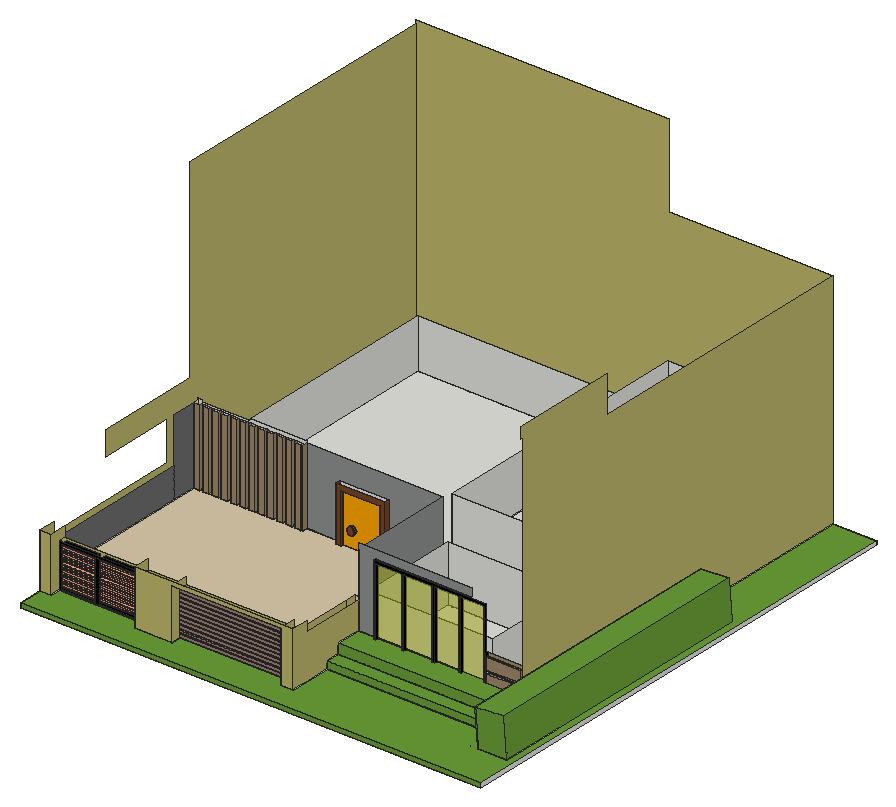
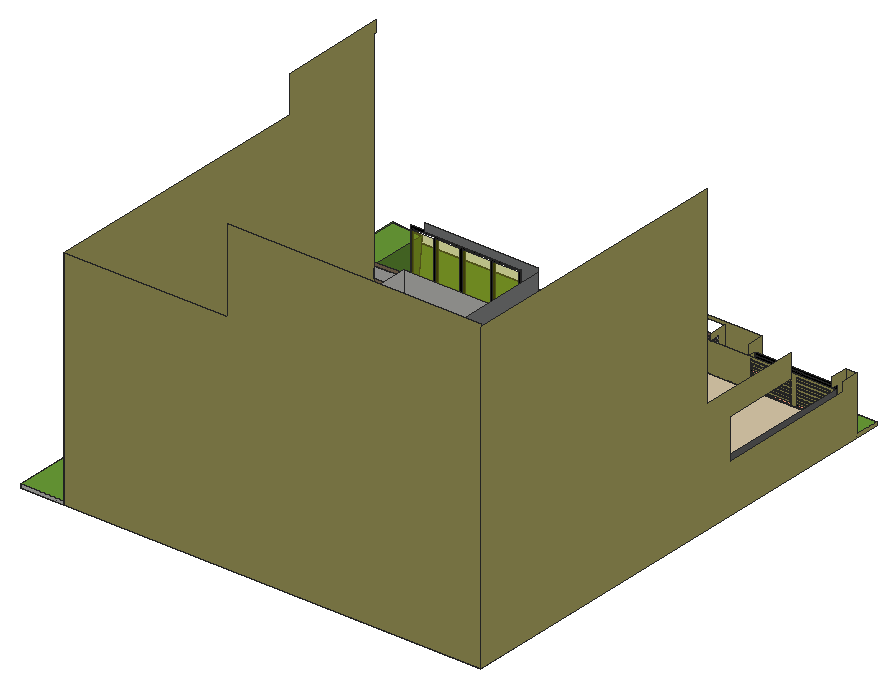
# SketchUp Ruby script. Lengths in inches.
U = 1.inch
M = Sketchup.active_model
def pt(a) = Geom::Point3d.new(a.map { |v| v * U })
def face(e, loops, mat)
  f = e.add_face(loops[0].map { |a| pt(a) })
  loops[1..].each { |l| e.add_face(l.map { |a| pt(a) }).erase! }
  f.material = f.back_material = mat if mat
  f
end
# faces: each face lists its corners as indices into pts; further lists are holes
def faces(e, pts, list, mat = nil) = list.each { |f| face(e, (f[0].is_a?(Array) ? f : [f]).map { |l| l.map { |i| pts[i] } }, mat) }
# xy, xz, yz: faces in a plane at the given z, y or x. An outline is a flat list of corners, or four numbers for a rectangle; further outlines are holes
def ring(l) = l.size == 4 ? [[l[0], l[1]], [l[2], l[1]], [l[2], l[3]], [l[0], l[3]]] : l.each_slice(2).to_a
def flat(e, list, mat, &to3) = list.each { |f| face(e, (f[0].is_a?(Array) ? f : [f]).map { |l| ring(l).map { |u, v| to3.(u, v) } }, mat) }
def xy(e, z, list, mat = nil) = flat(e, list, mat) { |x, y| [x, y, z] }
def xz(e, y, list, mat = nil) = flat(e, list, mat) { |x, z| [x, y, z] }
def yz(e, x, list, mat = nil) = flat(e, list, mat) { |y, z| [x, y, z] }
def lines(e, pts, list) = list.each { |a, b| e.add_line(pt(pts[a]), pt(pts[b])) }
# prism: a flat outline (further loops are holes) pulled along v
def prism(e, loops, v, mat = nil)
  f = face(e, loops, mat); d = Geom::Vector3d.new(v.map { |x| x * U })
  f.pushpull(f.normal.samedirection?(d) ? d.length : -d.length)
end
def box(e, o, s, mat = nil) = prism(e, [[o, [o[0] + s[0], o[1], o[2]], [o[0] + s[0], o[1] + s[1], o[2]], [o[0], o[1] + s[1], o[2]]]], [0, 0, s[2]], mat)
def at(x, y, z, deg = 0) = Geom::Transformation.translation(pt([x, y, z])) * Geom::Transformation.rotation(ORIGIN, Z_AXIS, deg.degrees)
def axes(o, x, y, z) = Geom::Transformation.new([*x, 0, *y, 0, *z, 0, *pt(o).to_a, 1])
def part(name) = M.definitions.add(name)
# library, detail: a bought-in or finely detailed component or shape, given as its bounding box
def library(name, o, s) = part(name).tap { |d| box(d.entities, o, s) }
def detail(e, o, s) = box(e.add_group.entities, o, s)
def put(e, d, t, mat = nil) = e.add_instance(d, t).tap { |i| i.material = mat if mat }
def group(e, t, mat = nil) = e.add_group.tap { |g| g.transformation = t; g.material = mat if mat }.entities
root = M.entities
M.materials.add("Niraj_Hair_Dark").color = [109, 109, 109]
M.materials.add("Niraj_Skin").color = [158, 128, 115]
M.materials.add("[0026_LightSalmon]").color = [255, 160, 122]
M.materials.add("[0035_Tan]").color = [158, 135, 105]
M.materials.add("[0038_Orange]").color = [255, 165, 0]
M.materials.add("[0057_DarkKhaki]").color = [189, 183, 107]
M.materials.add("[0137_Black]").color = [0, 0, 0]
M.materials.add("[Blacktop Old 02]").color = [143, 145, 145]
M.materials.add("[Field Square Tile]").color = [217, 201, 169]
M.materials.add("[Grass Dark Green]").color = [106, 157, 55]
M.materials.add("[Translucent Glass Gray]").color = [198, 206, 26]
M.materials["[Translucent Glass Gray]"].alpha = 0.5
M.materials.add("[Wood Veneer 01]").color = [120, 70, 37]
xy(root,0,[[3.5,0,3.5,42.8125,300.3,42.8125,300.3,30.8125,316.1875,30.8125,316.1875,0],[316.1875,0,518.75,42.8125],[518.75,0,572.19,42.8125],[300.3,30.8125,316.1875,42.8125],[3.5,42.8125,3.5,226.5,12.5,226.5,12.5,51.8125,307.1875,51.8125,307.1875,137.32,316.1875,137.32,316.1875,42.8125],
  [316.1875,42.8125,518.75,51.8125],[518.75,42.8125,518.75,51.8125,563.19,51.8125,563.19,611.5,572.19,611.5,572.19,42.8125],[12.5,51.8125,12.5,256.5,20.37,256.5,20.37,259.5,23.875,259.5,23.875,256.5,31.74,256.5,31.74,259.5,35.25,259.5,35.25,256.5,43.12,256.5,43.12,259.5,46.625,259.5,46.625,256.5,54.49,256.5,54.49,259.5,58,259.5,58,256.5,65.87,256.5,65.87,259.5,69.375,259.5,69.375,256.5,77.24,256.5,77.24,259.5,80.75,259.5,80.75,256.5,88.62,256.5,88.62,259.5,92.125,259.5,92.125,256.5,99.99,256.5,99.99,259.5,103.5,259.5,103.5,256.5,111.37,256.5,111.37,259.5,114.875,259.5,114.875,256.5,122.74,256.5,122.74,259.5,126.25,259.5,126.25,256.5,134.12,256.5,134.12,259.5,137.625,259.5,137.625,256.5,147.33,256.5,147.33,262.5,188.48,262.5,188.48,256.5,194.48,256.5,194.48,259.5,242.48,259.5,242.48,256.5,248.48,256.5,248.48,262.5,316.1875,262.5,316.1875,137.32,307.1875,137.32,307.1875,51.8125],[316.1875,51.8125,518.75,122.5],[518.75,51.8125,518.75,122.5,527.75,122.5,527.75,611.5,563.19,611.5,563.19,51.8125],
  [316.1875,122.5,518.75,131.5],[518.75,122.5,527.75,611.5],[[316.1875,131.5,316.1875,262.5,12.5,262.5,12.5,226.5,3.5,226.5,3.5,611.5,518.75,611.5,518.75,131.5],[12.5,268.5,316.1875,602.5],[322.1875,268.5,474.5,602.5],[322.1875,140.5,474.5,262.5]],[322.1875,140.5,474.5,262.5],[12.5,256.5,20.37,259.5],
  [23.875,256.5,31.74,259.5],[35.25,256.5,43.12,259.5],[46.625,256.5,54.49,259.5],[58,256.5,65.87,259.5],[69.375,256.5,77.24,259.5],
  [80.75,256.5,88.62,259.5],[92.125,256.5,99.99,259.5],[103.5,256.5,111.37,259.5],[114.875,256.5,122.74,259.5],[126.25,256.5,134.12,259.5],
  [137.625,256.5,145.49,259.5],[145.49,256.5,147.33,259.5],[188.48,256.5,194.48,262.5],[242.48,256.5,248.48,262.5],[12.5,259.5,147.33,262.5],
  [194.48,259.5,242.48,262.5],[12.5,268.5,316.1875,602.5],[322.1875,268.5,474.5,602.5]])
xy(root,1.66,[[119.91,30.8125,166.59,42.8125],[300.3,30.8125,316.1875,42.8125]])
xy(root,2.3125,[[316.1875,51.625,527.75,51.8125],[316.1875,51.8125,527.75,83.13],[316.1875,83.13,527.75,99.83],[316.1875,99.83,527.75,131.5]])
xy(root,4.9375,[[316.1875,122.5,518.75,131.5]])
xy(root,4.9375,[[3.5,0,572.19,0,572.19,611.5,518.75,611.5,518.75,83.13,527.75,83.13,527.75,51.8125,527.56,51.8125,527.75,51.8125,527.75,83.13,316.1875,83.13,316.1875,30.8125,300.3,30.8125,300.3,42.8125,166.59,42.8125,166.59,30.8125,119.91,30.8125,119.91,42.8125,17,42.8125,17,30.8125,3.5,30.8125]],"[Grass Dark Green]")
xy(root,5.11,[[20,42.8125,60.71,51.8125],[67.15,42.8125,116.91,51.8125]],"[0137_Black]")
xy(root,6.52,[[475.91,128.5,518.75,131.5]])
xy(root,6.74,[[166.59,40.8125,300.3,42.8125]])
xy(root,7.4375,[[67.15,42.8125,116.91,51.8125]])
xy(root,7.4375,[[20,42.8125,60.71,51.8125]],"[0026_LightSalmon]")
xy(root,8.93,[[20,42.8125,60.71,51.8125],[67.15,42.8125,116.91,51.8125]],"[0026_LightSalmon]")
xy(root,10,[[166.59,40.8125,300.3,42.8125]],"Niraj_Skin")
xy(root,11.25,[[20,42.8125,60.71,51.8125],[67.15,42.8125,116.91,51.8125]],"[0026_LightSalmon]")
xy(root,11.74,[[166.59,40.8125,300.3,42.8125]])
xy(root,12.74,[[20,42.8125,60.71,51.8125],[67.15,42.8125,116.91,51.8125]],"[0026_LightSalmon]")
xy(root,14.3125,[[316.1875,83.13,527.75,99.83]],"[Grass Dark Green]")
xy(root,15,[[166.59,40.8125,300.3,42.8125]],"Niraj_Skin")
xy(root,15.0625,[[20,42.8125,60.71,51.8125],[67.15,42.8125,116.91,51.8125]],"[0026_LightSalmon]")
xy(root,16.55,[[20,42.8125,60.71,51.8125],[67.15,42.8125,116.91,51.8125]],"[0026_LightSalmon]")
xy(root,16.74,[[166.59,40.8125,300.3,42.8125]],"Niraj_Skin")
xy(root,18.875,[[20,42.8125,60.71,51.8125],[67.15,42.8125,116.91,51.8125]],"[0026_LightSalmon]")
xy(root,19.34,[[337.16,128.5,475.91,131.5]])
xy(root,20,[[166.59,40.8125,300.3,42.8125]],"Niraj_Skin")
xy(root,20.36,[[20,42.8125,60.71,51.8125],[67.15,42.8125,116.91,51.8125]],"[0026_LightSalmon]")
xy(root,20.375,[[475.91,128.5,518.75,131.5]])
xy(root,21.74,[[166.59,40.8125,300.3,42.8125]],"Niraj_Skin")
xy(root,22.34,[[340.16,128.5,371.84,131.5],[374.84,128.5,409.66,131.5],[412.66,128.5,442.41,131.5],[445.41,128.5,472.91,131.5]])
xy(root,22.58,[[475.91,128.5,518.75,131.5]])
xy(root,22.6875,[[20,42.8125,60.71,51.8125],[67.15,42.8125,116.91,51.8125]],"[0026_LightSalmon]")
xy(root,22.75,[[12.5,51.8125,307.1875,51.8125,307.1875,137.32,316.1875,137.32,316.1875,262.5,248.48,262.5,248.48,256.5,242.48,256.5,242.48,259.5,194.48,259.5,194.48,256.5,188.48,256.5,188.48,262.5,147.33,262.5,147.33,256.5,137.625,256.5,137.625,259.5,134.12,259.5,134.12,256.5,126.25,256.5,126.25,259.5,122.74,259.5,122.74,256.5,114.875,256.5,114.875,259.5,111.37,259.5,111.37,256.5,103.5,256.5,103.5,259.5,99.99,259.5,99.99,256.5,92.125,256.5,92.125,259.5,88.62,259.5,88.62,256.5,80.75,256.5,80.75,259.5,77.24,259.5,77.24,256.5,69.375,256.5,69.375,259.5,65.87,259.5,65.87,256.5,58,256.5,58,259.5,54.49,259.5,54.49,256.5,46.625,256.5,46.625,259.5,43.12,259.5,43.12,256.5,35.25,256.5,35.25,259.5,31.74,259.5,31.74,256.5,23.875,256.5,23.875,259.5,20.37,259.5,20.37,256.5,12.5,256.5]],"[Field Square Tile]")
xy(root,24.18,[[20,42.8125,60.71,51.8125],[67.15,42.8125,116.91,51.8125]],"[0026_LightSalmon]")
xy(root,25,[[166.59,40.8125,300.3,42.8125]],"Niraj_Skin")
xy(root,26.3125,[[316.1875,99.83,527.75,131.5]],"[Grass Dark Green]")
xy(root,26.5,[[20,42.8125,60.71,51.8125],[67.15,42.8125,116.91,51.8125]],"[0026_LightSalmon]")
xy(root,26.74,[[166.59,40.8125,300.3,42.8125]],"Niraj_Skin")
xy(root,27.99,[[20,42.8125,60.71,51.8125],[67.15,42.8125,116.91,51.8125]],"[0026_LightSalmon]")
xy(root,30,[[166.59,40.8125,300.3,42.8125]],"Niraj_Skin")
xy(root,30.3125,[[20,42.8125,60.71,51.8125],[67.15,42.8125,116.91,51.8125]],"[0026_LightSalmon]")
xy(root,31.74,[[166.59,40.8125,300.3,42.8125]],"Niraj_Skin")
xy(root,31.8,[[20,42.8125,60.71,51.8125],[67.15,42.8125,116.91,51.8125]],"[0026_LightSalmon]")
xy(root,34.125,[[20,42.8125,60.71,51.8125],[67.15,42.8125,116.91,51.8125]],"[0026_LightSalmon]")
xy(root,35,[[166.59,40.8125,300.3,42.8125]],"Niraj_Skin")
xy(root,35.61,[[20,42.8125,60.71,51.8125],[67.15,42.8125,116.91,51.8125]],"[0026_LightSalmon]")
xy(root,36.4375,[[475.91,128.5,518.75,131.5]],"[0035_Tan]")
xy(root,36.74,[[166.59,40.8125,300.3,42.8125]],"Niraj_Skin")
xy(root,37.9375,[[20,42.8125,60.71,51.8125],[67.15,42.8125,116.91,51.8125]],"[0026_LightSalmon]")
xy(root,39.43,[[20,42.8125,60.71,51.8125],[67.15,42.8125,116.91,51.8125]],"[0026_LightSalmon]")
xy(root,40,[[166.59,40.8125,300.3,42.8125]],"Niraj_Skin")
xy(root,40.58,[[475.91,128.5,518.75,131.5]])
xy(root,41.74,[[166.59,40.8125,300.3,42.8125]],"Niraj_Skin")
xy(root,41.75,[[20,42.8125,60.71,51.8125],[67.15,42.8125,116.91,51.8125]],"[0026_LightSalmon]")
xy(root,43.24,[[20,42.8125,60.71,51.8125],[67.15,42.8125,116.91,51.8125]],"[0026_LightSalmon]")
xy(root,45,[[166.59,40.8125,300.3,42.8125]],"Niraj_Skin")
xy(root,45.5625,[[20,42.8125,60.71,51.8125],[67.15,42.8125,116.91,51.8125]],"[0026_LightSalmon]")
xy(root,46.74,[[166.59,40.8125,300.3,42.8125]],"Niraj_Skin")
xy(root,47.05,[[20,42.8125,60.71,51.8125],[67.15,42.8125,116.91,51.8125]],"[0026_LightSalmon]")
xy(root,49.375,[[20,42.8125,60.71,51.8125],[67.15,42.8125,116.91,51.8125]],"[0026_LightSalmon]")
xy(root,50,[[166.59,40.8125,300.3,42.8125]],"Niraj_Skin")
xy(root,50.86,[[20,42.8125,60.71,51.8125],[67.15,42.8125,116.91,51.8125]],"[0026_LightSalmon]")
xy(root,51.74,[[166.59,40.8125,300.3,42.8125]],"Niraj_Skin")
xy(root,53.1875,[[20,42.8125,60.71,51.8125],[67.15,42.8125,116.91,51.8125]],"[0026_LightSalmon]")
xy(root,54.3125,[[322.1875,268.5,474.5,602.5]])
xy(root,54.4375,[[475.91,128.5,518.75,131.5]],"[0035_Tan]")
xy(root,54.68,[[20,42.8125,60.71,51.8125],[67.15,42.8125,116.91,51.8125]],"[0026_LightSalmon]")
xy(root,55,[[166.59,40.8125,300.3,42.8125]],"Niraj_Skin")
xy(root,56.74,[[166.59,40.8125,300.3,42.8125]],"Niraj_Skin")
xy(root,57,[[20,42.8125,60.71,51.8125],[67.15,42.8125,116.91,51.8125]],"[0137_Black]")
xz(root,0,[[3.5,0,572.19,4.9375]],"[Grass Dark Green]")
xz(root,30.8125,[[300.3,0,316.1875,1.66],[119.91,1.66,166.59,2.3125],[300.3,1.66,316.1875,2.3125],[119.91,2.3125,166.59,4.9375],[300.3,2.3125,316.1875,4.9375]])
xz(root,30.8125,[[3.5,4.9375,17,72],[119.91,4.9375,166.59,4.9375,166.59,67.8125,300.3,67.8125,300.3,4.9375,316.1875,4.9375,316.1875,72,119.91,72]],"[0057_DarkKhaki]")
xz(root,40.8125,[[166.59,6.74,300.3,10],[166.59,11.74,300.3,15],[166.59,16.74,300.3,20],[166.59,21.74,300.3,25],[166.59,26.74,300.3,30],
  [166.59,31.74,300.3,35],[166.59,36.74,300.3,40],[166.59,41.74,300.3,45],[166.59,46.74,300.3,50],[166.59,51.74,300.3,55],
  [166.59,56.74,300.3,60]],"Niraj_Skin")
xz(root,42.8125,[[300.3,0,316.1875,1.66],[20,1.3,116.91,3.625],[166.59,1.74,300.3,4.9375],[166.59,4.9375,300.3,5],[166.59,6.74,300.3,10],
  [166.59,11.74,300.3,15],[166.59,16.74,300.3,20],[166.59,21.74,300.3,25],[166.59,26.74,300.3,30],[166.59,31.74,300.3,35],
  [166.59,36.74,300.3,40],[166.59,41.74,300.3,45],[166.59,46.74,300.3,50],[166.59,51.74,300.3,55]])
xz(root,42.8125,[[166.59,5,300.3,6.74],[166.59,10,300.3,11.74],[166.59,15,300.3,16.74],[166.59,20,300.3,21.74],[166.59,25,300.3,26.74],
  [166.59,30,300.3,31.74],[166.59,35,300.3,36.74],[166.59,40,300.3,41.74],[166.59,45,300.3,46.74],[166.59,50,300.3,51.74],
  [166.59,55,300.3,56.74]],"Niraj_Skin")
xz(root,42.8125,[[20,11.25,60.71,12.74],[67.15,11.25,116.91,12.74],[20,15.0625,60.71,16.55],[67.15,15.0625,116.91,16.55],[20,18.875,60.71,20.36],
  [67.15,18.875,116.91,20.36],[20,22.6875,60.71,24.18],[67.15,22.6875,116.91,24.18],[20,26.5,60.71,27.99],[67.15,26.5,116.91,27.99],
  [20,30.3125,60.71,31.8],[67.15,30.3125,116.91,31.8],[20,34.125,60.71,35.61],[67.15,34.125,116.91,35.61],[20,37.9375,60.71,39.43],
  [67.15,37.9375,116.91,39.43],[20,41.75,60.71,43.24],[67.15,41.75,116.91,43.24],[20,45.5625,60.71,47.05],[67.15,45.5625,116.91,47.05],
  [20,49.375,60.71,50.86],[67.15,49.375,116.91,50.86],[20,53.1875,60.71,54.68],[67.15,53.1875,116.91,54.68]],"[0026_LightSalmon]")
xz(root,42.8125,[[[17,4.9375,119.91,60],[20,5.11,20,7.4375,60.71,7.4375,60.71,8.93,20,8.93,20,57,116.91,57,116.91,8.93,67.15,8.93,67.15,7.4375,116.91,7.4375,116.91,5.11]],[60.71,5.11,67.15,57]],"[0137_Black]")
xz(root,51.8125,[[12.5,0,12.5,22.75,21.5,22.75,21.5,22.6875,20,22.6875,20,20.36,21.5,20.36,21.5,18.875,20,18.875,20,16.55,21.5,16.55,21.5,15.0625,20,15.0625,20,12.74,21.5,12.74,21.5,11.25,20,11.25,20,8.93,21.5,8.93,21.5,7.4375,20,7.4375,20,5.11,21.5,5.11,21.5,0],[[21.5,0,21.5,5.11,60.71,5.11,60.71,7.4375,21.5,7.4375,21.5,8.93,60.71,8.93,60.71,11.25,21.5,11.25,21.5,12.74,60.71,12.74,60.71,15.0625,21.5,15.0625,21.5,16.55,60.71,16.55,60.71,18.875,21.5,18.875,21.5,20.36,60.71,20.36,60.71,22.6875,21.5,22.6875,21.5,22.75,300.3,22.75,300.3,1.66,307.1875,1.66,307.1875,0],[67.15,16.55,116.91,18.875],[67.15,5.11,116.91,7.4375],[67.15,20.36,116.91,22.6875],[67.15,12.74,116.91,15.0625],[67.15,8.93,116.91,11.25]],[316.1875,0,563.19,2.3125],[300.3,1.66,307.1875,22.75],[527.75,2.3125,527.75,4.9375,527.56,4.9375],
  [527.75,2.3125,563.19,2.3125,563.19,4.9375],[527.75,2.3125,563.19,4.9375,527.75,4.9375],[20,5.11,21.5,7.4375],[21.5,5.11,60.71,7.4375],[20,8.93,21.5,11.25],
  [21.5,8.93,60.71,11.25],[20,12.74,21.5,15.0625],[21.5,12.74,60.71,15.0625],[20,16.55,21.5,18.875],[21.5,16.55,60.71,18.875],
  [20,20.36,21.5,22.6875],[21.5,20.36,60.71,22.6875]])
xz(root,51.8125,[[[12.5,22.75,307.1875,60],[67.15,54.68,116.91,57],[67.15,50.86,116.91,53.1875],[67.15,47.05,116.91,49.375],[67.15,43.24,116.91,45.5625],[67.15,31.8,116.91,34.125],[67.15,27.99,116.91,30.3125],[67.15,24.18,116.91,26.5],[67.15,39.43,116.91,41.75],[67.15,35.61,116.91,37.9375],[20,54.68,60.71,57],[20,50.86,60.71,53.1875],[20,47.05,60.71,49.375],[20,43.24,60.71,45.5625],[20,24.18,60.71,26.5],[20,27.99,60.71,30.3125],[20,31.8,60.71,34.125],[20,39.43,60.71,41.75],[20,35.61,60.71,37.9375]]],"[0057_DarkKhaki]")
xz(root,51.8125,[[527.56,4.9375,563.19,4.9375,559.65,52.81,524.2,50.18]],"[Grass Dark Green]")
xz(root,83.13,[[316.1875,2.3125,527.75,4.9375]])
xz(root,83.13,[[316.1875,4.9375,527.75,14.3125]],"[Grass Dark Green]")
xz(root,99.83,[[316.1875,2.3125,527.75,14.3125]])
xz(root,99.83,[[316.1875,14.3125,527.75,26.3125]],"[Grass Dark Green]")
xz(root,122.5,[[316.1875,0,527.75,4.9375]])
xz(root,128.5,[[475.91,6.52,518.75,20.375]])
xz(root,128.5,[[475.91,22.58,518.75,36.4375],[475.91,40.58,518.75,54.4375]],"[0035_Tan]")
xz(root,128.5,[[[337.16,19.34,475.91,113.09],[374.84,22.34,409.66,110.09],[340.16,22.34,371.84,110.09],[412.66,22.34,442.41,110.09],[445.41,22.34,472.91,110.09]]],"[0137_Black]")
xz(root,131.5,[[316.1875,0,518.75,1.66],[316.1875,1.66,518.75,2.3125],[316.1875,2.3125,518.75,4.9375],[518.75,2.3125,527.75,26.3125],[316.1875,4.9375,316.1875,26.3125,337.16,26.3125,337.16,19.34,475.91,19.34,475.91,6.52,518.75,6.52,518.75,4.9375],
  [475.91,6.52,518.75,20.375],[337.16,19.34,337.16,22.58,340.16,22.58,340.16,22.34,371.84,22.34,371.84,22.58,374.84,22.58,374.84,22.34,409.66,22.34,409.66,22.58,412.66,22.58,412.66,22.34,442.41,22.34,442.41,22.58,445.41,22.58,445.41,22.34,472.91,22.34,472.91,22.58,475.91,22.58,475.91,19.34],[337.16,19.34,475.91,22.58],[475.91,20.375,518.75,22.58],[340.16,22.34,371.84,22.58],
  [374.84,22.34,409.66,22.58],[412.66,22.34,442.41,22.58],[445.41,22.34,472.91,22.58],[337.16,22.58,340.16,26.3125],[340.16,22.58,371.84,26.3125],
  [371.84,22.58,374.84,26.3125],[374.84,22.58,409.66,26.3125],[409.66,22.58,412.66,26.3125],[412.66,22.58,442.41,26.3125],[442.41,22.58,445.41,26.3125],
  [445.41,22.58,472.91,26.3125],[472.91,22.58,475.91,26.3125],[475.91,22.58,518.75,26.3125],[337.16,26.3125,340.16,36.4375],[371.84,26.3125,374.84,36.4375],
  [409.66,26.3125,412.66,36.4375],[442.41,26.3125,445.41,36.4375],[472.91,26.3125,475.91,36.4375],[475.91,26.3125,518.75,36.4375],[337.16,36.4375,340.16,40.58],
  [371.84,36.4375,374.84,40.58],[409.66,36.4375,412.66,40.58],[442.41,36.4375,445.41,40.58],[472.91,36.4375,475.91,40.58],[337.16,40.58,340.16,54.4375],
  [371.84,40.58,374.84,54.4375],[409.66,40.58,412.66,54.4375],[442.41,40.58,445.41,54.4375],[472.91,40.58,475.91,54.4375],[475.91,40.58,518.75,54.4375],
  [337.16,54.4375,340.16,58.58],[371.84,54.4375,374.84,58.58],[409.66,54.4375,412.66,58.58],[442.41,54.4375,445.41,58.58],[472.91,54.4375,475.91,58.58]])
xz(root,131.5,[[475.91,36.4375,518.75,40.58],[475.91,54.4375,518.75,58.58]],"[0035_Tan]")
xz(root,131.5,[[316.1875,26.3125,337.16,26.3125,337.16,113.09,456.23,113.09,456.23,123,316.1875,123]],"[Blacktop Old 02]")
xz(root,131.5,[[340.16,26.3125,371.84,110.09],[374.84,26.3125,409.66,110.09],[412.66,26.3125,442.41,110.09],[445.41,26.3125,472.91,110.09]],"[Translucent Glass Gray]")
xz(root,137.32,[[307.1875,0,316.1875,22.75],[307.1875,22.75,316.1875,60]])
xz(root,140.5,[[322.1875,0,474.5,68.75]])
xz(root,256.5,[[12.5,0,20.37,22.75],[23.875,0,31.74,22.75],[35.25,0,43.12,22.75],[46.625,0,54.49,22.75],[58,0,65.87,22.75],
  [69.375,0,77.24,22.75],[80.75,0,88.62,22.75],[92.125,0,99.99,22.75],[103.5,0,111.37,22.75],[114.875,0,122.74,22.75],
  [126.25,0,134.12,22.75],[137.625,0,145.49,22.75],[145.49,0,147.33,22.75],[188.48,0,194.48,22.75],[242.48,0,248.48,22.75]])
xz(root,256.5,[[12.5,22.75,20.37,117.125],[23.875,22.75,31.74,117.125],[35.25,22.75,43.12,117.125],[46.625,22.75,54.49,117.125],[58,22.75,65.87,117.125],
  [69.375,22.75,77.24,117.125],[80.75,22.75,88.62,117.125],[92.125,22.75,99.99,117.125],[103.5,22.75,111.37,117.125],[114.875,22.75,122.74,117.125],
  [126.25,22.75,134.12,117.125],[137.625,22.75,145.49,117.125],[145.49,22.75,147.33,117.125]],"[0035_Tan]")
xz(root,256.5,[[188.48,22.75,194.48,22.75,194.48,84,242.48,84,242.48,22.75,248.48,22.75,248.48,90,188.48,90],[206.5,37.91,207.72,38.07,208.85,38.54,209.82,39.28,210.5625,40.25,211.03,41.38,211.19,42.6,211.03,43.81,210.5625,44.94,209.82,45.91,208.85,46.66,207.72,47.125,206.5,47.28,205.29,47.125,204.16,46.66,203.19,45.91,202.44,44.94,201.98,43.81,201.82,42.6,201.98,41.38,202.44,40.25,203.19,39.28,204.16,38.54,205.29,38.07]],"[Wood Veneer 01]")
xz(root,259.5,[[20.37,0,23.875,22.75],[23.875,0,31.74,117.125],[31.74,0,35.25,22.75],[35.25,0,43.12,117.125],[43.12,0,46.625,22.75],
  [46.625,0,54.49,117.125],[54.49,0,58,22.75],[58,0,65.87,117.125],[65.87,0,69.375,22.75],[69.375,0,77.24,117.125],
  [77.24,0,80.75,22.75],[80.75,0,88.62,117.125],[88.62,0,92.125,22.75],[92.125,0,99.99,117.125],[99.99,0,103.5,22.75],
  [103.5,0,111.37,117.125],[111.37,0,114.875,22.75],[114.875,0,122.74,117.125],[122.74,0,126.25,22.75],[126.25,0,134.12,117.125],
  [134.12,0,137.625,22.75],[137.625,0,145.49,117.125],[194.48,0,242.48,22.75],[206.5,37.91,205.29,38.07,204.16,38.54,203.19,39.28,202.44,40.25,201.98,41.38,201.82,42.6,201.98,43.81,202.44,44.94,203.19,45.91,204.16,46.66,205.29,47.125,206.5,47.28,207.72,47.125,208.85,46.66,209.82,45.91,210.5625,44.94,211.03,43.81,211.19,42.6,211.03,41.38,210.5625,40.25,209.82,39.28,208.85,38.54,207.72,38.07]])
xz(root,259.5,[[20.37,22.75,23.875,117.125],[31.74,22.75,35.25,117.125],[43.12,22.75,46.625,117.125],[54.49,22.75,58,117.125],[65.87,22.75,69.375,117.125],
  [77.24,22.75,80.75,117.125],[88.62,22.75,92.125,117.125],[99.99,22.75,103.5,117.125],[111.37,22.75,114.875,117.125],[122.74,22.75,126.25,117.125],
  [134.12,22.75,137.625,117.125]],"[0035_Tan]")
xz(root,259.5,[[[194.48,22.75,242.48,84],[206.5,37.91,205.29,38.07,204.16,38.54,203.19,39.28,202.44,40.25,201.98,41.38,201.82,42.6,201.98,43.81,202.44,44.94,203.19,45.91,204.16,46.66,205.29,47.125,206.5,47.28,207.72,47.125,208.85,46.66,209.82,45.91,210.5625,44.94,211.03,43.81,211.19,42.6,211.03,41.38,210.5625,40.25,209.82,39.28,208.85,38.54,207.72,38.07]]],"[0038_Orange]")
xz(root,262.5,[[12.5,0,12.5,120,18.33,120,18.33,117,78.33,117,78.33,120,147.33,120,147.33,0],[147.33,0,188.48,22.75],[188.48,0,188.48,90,248.48,90,248.48,0,242.48,0,242.48,84,194.48,84,194.48,0],[194.48,0,242.48,84],[248.48,0,316.1875,22.75],
  [322.1875,0,474.5,68.75]])
xz(root,262.5,[[147.33,22.75,188.48,22.75,188.48,90,248.48,90,248.48,22.75,316.1875,22.75,316.1875,117.125,147.33,117.125]],"[Blacktop Old 02]")
xz(root,268.5,[[12.5,0,316.1875,61.1875],[322.1875,0,474.5,54.3125],[322.1875,54.3125,474.5,120]])
xz(root,399.65,[[527.75,2.3125,524.2,50.18,559.65,52.81,563.19,4.9375]])
xz(root,602.5,[[12.5,0,316.1875,61.1875],[322.1875,0,474.5,54.3125],[322.1875,54.3125,474.5,120]])
xz(root,611.5,[[518.75,0,572.19,4.9375]])
xz(root,611.5,[[3.5,0,3.5,381.875,316.1875,381.875,316.1875,279,518.75,279,518.75,0]],"[0057_DarkKhaki]")
yz(root,3.5,[[0,0,0,4.9375,30.8125,4.9375,30.8125,72,51.8125,72,51.8125,60,226.5,60,226.5,109.4375,131.5,109.4375,131.5,139.125,262.5,139.125,262.5,377.89,611.5,377.89,611.5,0]],"[0057_DarkKhaki]")
yz(root,12.5,[[51.8125,0,226.5,22.75],[226.5,0,256.5,22.75],[256.5,0,262.5,117.125],[268.5,0,602.5,61.1875]])
yz(root,12.5,[[51.8125,22.75,226.5,60],[226.5,22.75,256.5,117.125]],"Niraj_Hair_Dark")
yz(root,17,[[30.8125,1.66,42.8125,4.9375]])
yz(root,17,[[30.8125,4.9375,42.8125,4.9375,42.8125,60,51.8125,60,51.8125,72,30.8125,72]],"[0057_DarkKhaki]")
yz(root,20,[[42.8125,5.11,51.8125,7.4375],[42.8125,8.93,51.8125,11.25],[42.8125,12.74,51.8125,15.0625],[42.8125,16.55,51.8125,18.875],[42.8125,20.36,51.8125,22.6875],
  [42.8125,24.18,51.8125,26.5],[42.8125,27.99,51.8125,30.3125],[42.8125,31.8,51.8125,34.125],[42.8125,35.61,51.8125,37.9375],[42.8125,39.43,51.8125,41.75],
  [42.8125,43.24,51.8125,45.5625],[42.8125,47.05,51.8125,49.375],[42.8125,50.86,51.8125,53.1875],[42.8125,54.68,51.8125,57]],"[0137_Black]")
yz(root,20.37,[[256.5,0,259.5,22.75]])
yz(root,20.37,[[256.5,22.75,259.5,117.125]],"[0035_Tan]")
yz(root,23.875,[[256.5,0,259.5,22.75]])
yz(root,23.875,[[256.5,22.75,259.5,117.125]],"[0035_Tan]")
yz(root,31.74,[[256.5,0,259.5,22.75]])
yz(root,31.74,[[256.5,22.75,259.5,117.125]],"[0035_Tan]")
yz(root,35.25,[[256.5,0,259.5,22.75]])
yz(root,35.25,[[256.5,22.75,259.5,117.125]],"[0035_Tan]")
yz(root,43.12,[[256.5,0,259.5,22.75]])
yz(root,43.12,[[256.5,22.75,259.5,117.125]],"[0035_Tan]")
yz(root,46.625,[[256.5,0,259.5,22.75]])
yz(root,46.625,[[256.5,22.75,259.5,117.125]],"[0035_Tan]")
yz(root,54.49,[[256.5,0,259.5,22.75]])
yz(root,54.49,[[256.5,22.75,259.5,117.125]],"[0035_Tan]")
yz(root,58,[[256.5,0,259.5,22.75]])
yz(root,58,[[256.5,22.75,259.5,117.125]],"[0035_Tan]")
yz(root,60.71,[[42.8125,5.11,51.8125,7.4375],[42.8125,8.93,51.8125,11.25],[42.8125,12.74,51.8125,15.0625],[42.8125,16.55,51.8125,18.875],[42.8125,20.36,51.8125,22.6875],
  [42.8125,24.18,51.8125,26.5],[42.8125,27.99,51.8125,30.3125],[42.8125,31.8,51.8125,34.125],[42.8125,35.61,51.8125,37.9375],[42.8125,39.43,51.8125,41.75],
  [42.8125,43.24,51.8125,45.5625],[42.8125,47.05,51.8125,49.375],[42.8125,50.86,51.8125,53.1875],[42.8125,54.68,51.8125,57]],"[0137_Black]")
yz(root,65.87,[[256.5,0,259.5,22.75]])
yz(root,65.87,[[256.5,22.75,259.5,117.125]],"[0035_Tan]")
yz(root,67.15,[[42.8125,5.11,51.8125,7.4375],[42.8125,8.93,51.8125,11.25],[42.8125,12.74,51.8125,15.0625],[42.8125,16.55,51.8125,18.875],[42.8125,20.36,51.8125,22.6875],
  [42.8125,24.18,51.8125,26.5],[42.8125,27.99,51.8125,30.3125],[42.8125,31.8,51.8125,34.125],[42.8125,35.61,51.8125,37.9375],[42.8125,39.43,51.8125,41.75],
  [42.8125,43.24,51.8125,45.5625],[42.8125,47.05,51.8125,49.375],[42.8125,50.86,51.8125,53.1875],[42.8125,54.68,51.8125,57]],"[0137_Black]")
yz(root,69.375,[[256.5,0,259.5,22.75]])
yz(root,69.375,[[256.5,22.75,259.5,117.125]],"[0035_Tan]")
yz(root,77.24,[[256.5,0,259.5,22.75]])
yz(root,77.24,[[256.5,22.75,259.5,117.125]],"[0035_Tan]")
yz(root,80.75,[[256.5,0,259.5,22.75]])
yz(root,80.75,[[256.5,22.75,259.5,117.125]],"[0035_Tan]")
yz(root,88.62,[[256.5,0,259.5,22.75]])
yz(root,88.62,[[256.5,22.75,259.5,117.125]],"[0035_Tan]")
yz(root,92.125,[[256.5,0,259.5,22.75]])
yz(root,92.125,[[256.5,22.75,259.5,117.125]],"[0035_Tan]")
yz(root,99.99,[[256.5,0,259.5,22.75]])
yz(root,99.99,[[256.5,22.75,259.5,117.125]],"[0035_Tan]")
yz(root,103.5,[[256.5,0,259.5,22.75]])
yz(root,103.5,[[256.5,22.75,259.5,117.125]],"[0035_Tan]")
yz(root,111.37,[[256.5,0,259.5,22.75]])
yz(root,111.37,[[256.5,22.75,259.5,117.125]],"[0035_Tan]")
yz(root,114.875,[[256.5,0,259.5,22.75]])
yz(root,114.875,[[256.5,22.75,259.5,117.125]],"[0035_Tan]")
yz(root,116.91,[[42.8125,5.11,51.8125,7.4375],[42.8125,8.93,51.8125,11.25],[42.8125,12.74,51.8125,15.0625],[42.8125,16.55,51.8125,18.875],[42.8125,20.36,51.8125,22.6875],
  [42.8125,24.18,51.8125,26.5],[42.8125,27.99,51.8125,30.3125],[42.8125,31.8,51.8125,34.125],[42.8125,35.61,51.8125,37.9375],[42.8125,39.43,51.8125,41.75],
  [42.8125,43.24,51.8125,45.5625],[42.8125,47.05,51.8125,49.375],[42.8125,50.86,51.8125,53.1875],[42.8125,54.68,51.8125,57]],"[0137_Black]")
yz(root,119.91,[[30.8125,1.66,42.8125,4.9375]])
yz(root,119.91,[[30.8125,4.9375,30.8125,72,51.8125,72,51.8125,60,42.8125,60,42.8125,4.9375]],"[0057_DarkKhaki]")
yz(root,122.74,[[256.5,0,259.5,22.75]])
yz(root,122.74,[[256.5,22.75,259.5,117.125]],"[0035_Tan]")
yz(root,126.25,[[256.5,0,259.5,22.75]])
yz(root,126.25,[[256.5,22.75,259.5,117.125]],"[0035_Tan]")
yz(root,134.12,[[256.5,0,259.5,22.75]])
yz(root,134.12,[[256.5,22.75,259.5,117.125]],"[0035_Tan]")
yz(root,137.625,[[256.5,0,259.5,22.75]])
yz(root,137.625,[[256.5,22.75,259.5,117.125]],"[0035_Tan]")
yz(root,145.49,[[256.5,0,259.5,117.125]])
yz(root,147.33,[[256.5,0,259.5,22.75],[259.5,0,262.5,22.75]])
yz(root,147.33,[[256.5,22.75,262.5,117.125]],"[0035_Tan]")
yz(root,166.59,[[30.8125,1.66,42.8125,4.9375],[40.8125,6.74,42.8125,10],[40.8125,11.74,42.8125,15],[40.8125,16.74,42.8125,20],[40.8125,21.74,42.8125,25],
  [40.8125,26.74,42.8125,30],[40.8125,31.74,42.8125,35],[40.8125,36.74,42.8125,40],[40.8125,41.74,42.8125,45],[40.8125,46.74,42.8125,50],
  [40.8125,51.74,42.8125,55],[40.8125,56.74,42.8125,60]])
yz(root,166.59,[[30.8125,4.9375,42.8125,4.9375,42.8125,6.74,40.8125,6.74,40.8125,10,42.8125,10,42.8125,11.74,40.8125,11.74,40.8125,15,42.8125,15,42.8125,16.74,40.8125,16.74,40.8125,20,42.8125,20,42.8125,21.74,40.8125,21.74,40.8125,25,42.8125,25,42.8125,26.74,40.8125,26.74,40.8125,30,42.8125,30,42.8125,31.74,40.8125,31.74,40.8125,35,42.8125,35,42.8125,36.74,40.8125,36.74,40.8125,40,42.8125,40,42.8125,41.74,40.8125,41.74,40.8125,45,42.8125,45,42.8125,46.74,40.8125,46.74,40.8125,50,42.8125,50,42.8125,51.74,40.8125,51.74,40.8125,55,42.8125,55,42.8125,56.74,40.8125,56.74,40.8125,60,51.8125,60,51.8125,67.8125,30.8125,67.8125]],"[0057_DarkKhaki]")
yz(root,188.48,[[256.5,0,259.5,22.75],[259.5,0,262.5,22.75]])
yz(root,188.48,[[256.5,22.75,262.5,90]],"[Wood Veneer 01]")
yz(root,194.48,[[256.5,0,259.5,22.75],[259.5,0,262.5,84]])
yz(root,194.48,[[256.5,22.75,259.5,84]],"[Wood Veneer 01]")
yz(root,242.48,[[256.5,0,259.5,22.75],[259.5,0,262.5,84]])
yz(root,242.48,[[256.5,22.75,259.5,84]],"[Wood Veneer 01]")
yz(root,248.48,[[256.5,0,262.5,22.75]])
yz(root,248.48,[[256.5,22.75,262.5,90]],"[Wood Veneer 01]")
yz(root,300.3,[[30.8125,0,42.8125,1.66],[30.8125,1.66,42.8125,4.9375],[40.8125,6.74,42.8125,10],[40.8125,11.74,42.8125,15],[40.8125,16.74,42.8125,20],
  [40.8125,21.74,42.8125,25],[40.8125,26.74,42.8125,30],[40.8125,31.74,42.8125,35],[40.8125,36.74,42.8125,40],[40.8125,41.74,42.8125,45],
  [40.8125,46.74,42.8125,50],[40.8125,51.74,42.8125,55],[40.8125,56.74,42.8125,60]])
yz(root,300.3,[[30.8125,4.9375,30.8125,67.8125,51.8125,67.8125,51.8125,60,40.8125,60,40.8125,56.74,42.8125,56.74,42.8125,55,40.8125,55,40.8125,51.74,42.8125,51.74,42.8125,50,40.8125,50,40.8125,46.74,42.8125,46.74,42.8125,45,40.8125,45,40.8125,41.74,42.8125,41.74,42.8125,40,40.8125,40,40.8125,36.74,42.8125,36.74,42.8125,35,40.8125,35,40.8125,31.74,42.8125,31.74,42.8125,30,40.8125,30,40.8125,26.74,42.8125,26.74,42.8125,25,40.8125,25,40.8125,21.74,42.8125,21.74,42.8125,20,40.8125,20,40.8125,16.74,42.8125,16.74,42.8125,15,40.8125,15,40.8125,11.74,42.8125,11.74,42.8125,10,40.8125,10,40.8125,6.74,42.8125,6.74,42.8125,4.9375]],"[0057_DarkKhaki]")
yz(root,307.1875,[[51.8125,0,122.5,22.75],[122.5,0,137.32,22.75]])
yz(root,307.1875,[[51.8125,22.75,122.5,60],[122.5,22.75,137.32,60]],"[0057_DarkKhaki]")
yz(root,316.1875,[[30.8125,0,42.8125,1.66],[42.8125,0,51.8125,1.66],[51.8125,0,122.5,1.66],[122.5,0,131.5,1.66],[131.5,0,137.32,60],
  [137.32,0,140.5,22.75],[140.5,0,262.5,22.75],[268.5,0,602.5,61.1875],[30.8125,1.66,42.8125,2.3125],[42.8125,1.66,51.8125,2.3125],
  [51.8125,1.66,122.5,2.3125],[122.5,1.66,131.5,2.3125],[30.8125,2.3125,42.8125,4.9375],[42.8125,2.3125,51.625,4.9375],[51.625,2.3125,51.8125,4.9375],
  [51.8125,2.3125,83.13,4.9375],[83.13,2.3125,99.83,4.9375],[99.83,2.3125,122.5,4.9375],[122.5,2.3125,131.5,4.9375],[83.13,4.9375,99.83,14.3125],
  [99.83,4.9375,122.5,26.3125],[122.5,4.9375,131.5,26.3125]])
yz(root,316.1875,[[30.8125,4.9375,83.13,4.9375,83.13,14.3125,99.83,14.3125,99.83,26.3125,131.5,26.3125,131.5,60,51.8125,60,51.8125,72,30.8125,72]],"[0057_DarkKhaki]")
yz(root,316.1875,[[137.32,22.75,137.32,60,131.5,60,131.5,117.125,262.5,117.125,262.5,22.75]],"[Blacktop Old 02]")
yz(root,322.1875,[[140.5,0,262.5,68.75],[268.5,0,602.5,54.3125],[268.5,54.3125,602.5,120]])
yz(root,337.16,[[128.5,19.34,131.5,113.09]],"[0137_Black]")
yz(root,340.16,[[128.5,22.34,131.5,110.09]],"[0137_Black]")
yz(root,371.84,[[128.5,22.34,131.5,110.09]],"[0137_Black]")
yz(root,374.84,[[128.5,22.34,131.5,110.09]],"[0137_Black]")
yz(root,409.66,[[128.5,22.34,131.5,110.09]],"[0137_Black]")
yz(root,412.66,[[128.5,22.34,131.5,110.09]],"[0137_Black]")
yz(root,442.41,[[128.5,22.34,131.5,110.09]],"[0137_Black]")
yz(root,445.41,[[128.5,22.34,131.5,110.09]],"[0137_Black]")
yz(root,472.91,[[128.5,22.34,131.5,110.09]],"[0137_Black]")
yz(root,474.5,[[140.5,0,262.5,68.75],[268.5,0,602.5,54.3125],[268.5,54.3125,602.5,120]])
yz(root,475.91,[[128.5,6.52,131.5,19.34],[128.5,19.34,131.5,20.375],[128.5,20.375,131.5,22.58],[128.5,22.58,131.5,36.4375],[128.5,40.58,131.5,54.4375]])
yz(root,475.91,[[128.5,36.4375,131.5,40.58],[128.5,54.4375,131.5,58.58]],"[0137_Black]")
yz(root,518.75,[[131.5,0,611.5,1.66],[131.5,1.66,611.5,2.3125],[131.5,2.3125,611.5,4.9375],[128.5,6.52,131.5,20.375],[128.5,22.58,131.5,36.4375]])
yz(root,518.75,[[128.5,40.58,131.5,54.4375]],"[0035_Tan]")
yz(root,518.75,[[131.5,4.9375,611.5,4.9375,611.5,279,262.5,279,262.5,324.4375,128.5,324.4375,128.5,310.58,131.5,310.58]],"[0057_DarkKhaki]")
yz(root,527.75,[[122.5,0,131.5,2.3125],[51.8125,2.3125,83.13,4.9375],[83.13,2.3125,99.83,14.3125],[99.83,2.3125,122.5,26.3125],[122.5,2.3125,131.5,4.9375],
  [122.5,4.9375,131.5,26.3125]])
yz(root,563.19,[[51.8125,0,131.5,2.3125],[51.8125,2.3125,131.5,4.9375]])
yz(root,572.19,[[0,0,611.5,4.9375]])
p = [[527.75,51.8125,2.3125],[527.56,51.8125,4.9375],[527.56,51.625,4.9375],[527.75,51.625,2.3125],[527.75,399.65,2.3125],[527.75,131.5,2.3125],
  [527.75,122.5,2.3125],[527.75,99.83,2.3125],[527.75,83.13,2.3125],[524.2,51.8125,50.18],[524.2,399.65,50.18],[563.19,51.8125,4.9375],
  [563.19,131.5,4.9375],[563.19,399.65,4.9375],[559.65,399.65,52.81],[559.65,51.8125,52.81],[205.29,259.5,38.07],[206.5,259.5,37.91],
  [206.5,256.5,37.91],[205.29,256.5,38.07],[207.72,259.5,38.07],[207.72,256.5,38.07],[204.16,259.5,38.54],[204.16,256.5,38.54],
  [208.85,259.5,38.54],[208.85,256.5,38.54],[203.19,259.5,39.28],[203.19,256.5,39.28],[209.82,259.5,39.28],[209.82,256.5,39.28],
  [202.44,259.5,40.25],[202.44,256.5,40.25],[210.5625,259.5,40.25],[210.5625,256.5,40.25],[201.98,259.5,41.38],[201.98,256.5,41.38],
  [211.03,259.5,41.38],[211.03,256.5,41.38],[201.82,259.5,42.6],[201.82,256.5,42.6],[211.19,259.5,42.6],[211.19,256.5,42.6],
  [201.98,259.5,43.81],[201.98,256.5,43.81],[211.03,259.5,43.81],[211.03,256.5,43.81],[202.44,259.5,44.94],[202.44,256.5,44.94],
  [210.5625,259.5,44.94],[210.5625,256.5,44.94],[203.19,259.5,45.91],[203.19,256.5,45.91],[209.82,259.5,45.91],[209.82,256.5,45.91],
  [204.16,259.5,46.66],[204.16,256.5,46.66],[208.85,259.5,46.66],[208.85,256.5,46.66],[205.29,259.5,47.125],[205.29,256.5,47.125],
  [207.72,259.5,47.125],[207.72,256.5,47.125],[206.5,259.5,47.28],[206.5,256.5,47.28],[149,259.5,0],[156.87,259.5,0],
  [160.375,259.5,0],[168.24,259.5,0],[171.75,259.5,0],[179.62,259.5,0],[183.125,259.5,0],[188.48,259.5,0],
  [190.99,259.5,0],[-85.19,42.8125,0],[-85.19,42.8125,2.3125],[527.75,611.5,2.3125],[300.3,51.8125,1.66],[300.3,42.8125,1.66],
  [307.1875,51.8125,1.66],[316.1875,51.8125,1.66],[119.91,30.8125,2.3125],[17,30.8125,2.3125],[17,30.8125,1.66],[3.5,30.8125,1.66],
  [116.91,42.8125,7.9375],[116.91,42.8125,8.93],[20,42.8125,8.93],[20,42.8125,7.9375],[518.75,51.8125,4.9375],[518.75,51.625,4.9375]]
faces(root,p,[[0,1,2,3]])
faces(root,p,[[4,5,6,7,8,0,1,9,10],[11,12,13,14,15],[15,14,10,9]],"[Grass Dark Green]")
faces(root,p,[[16,17,18,19],[17,20,21,18],[22,16,19,23],[20,24,25,21],[26,22,23,27],[24,28,29,25],[30,26,27,31],[28,32,33,29],
  [34,30,31,35],[32,36,37,33],[38,34,35,39],[36,40,41,37],[42,38,39,43],[40,44,45,41],[46,42,43,47],[44,48,49,45],
  [50,46,47,51],[48,52,53,49],[54,50,51,55],[52,56,57,53],[58,54,55,59],[56,60,61,57],[62,58,59,63],[60,62,63,61]],"[Wood Veneer 01]")
lines(root,p,[[64,65],[66,67],[68,69],[70,71],[71,72],[73,74],[75,4],[76,77],[78,79],[80,81],[82,83],[84,85],
  [86,87],[88,89]])
